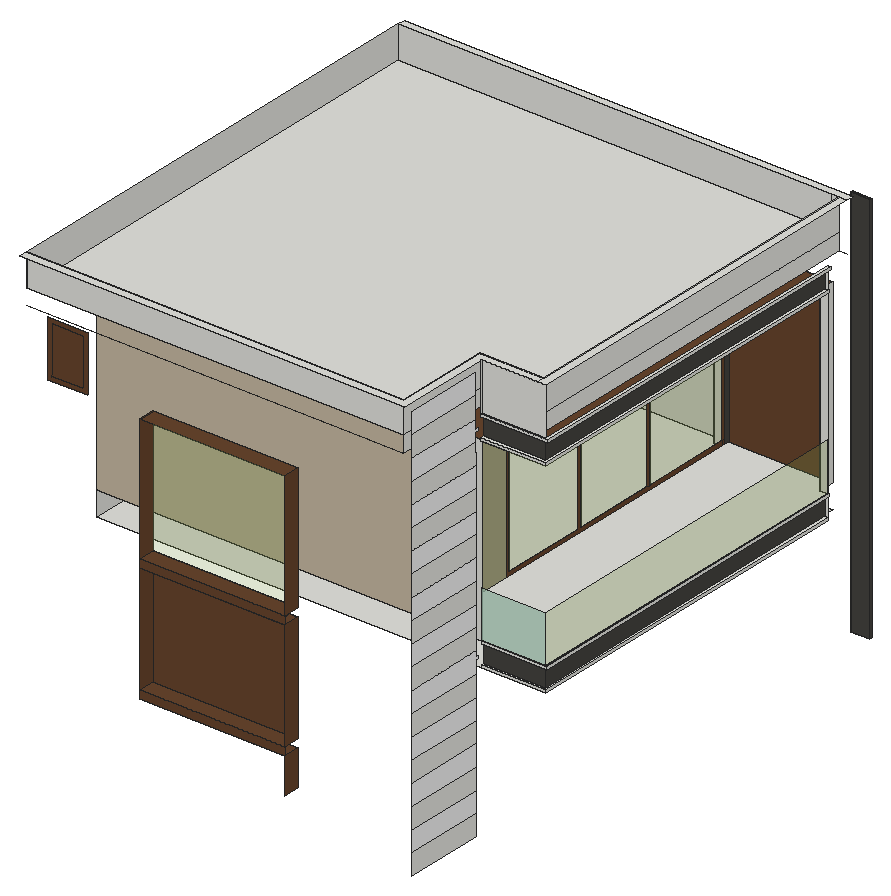
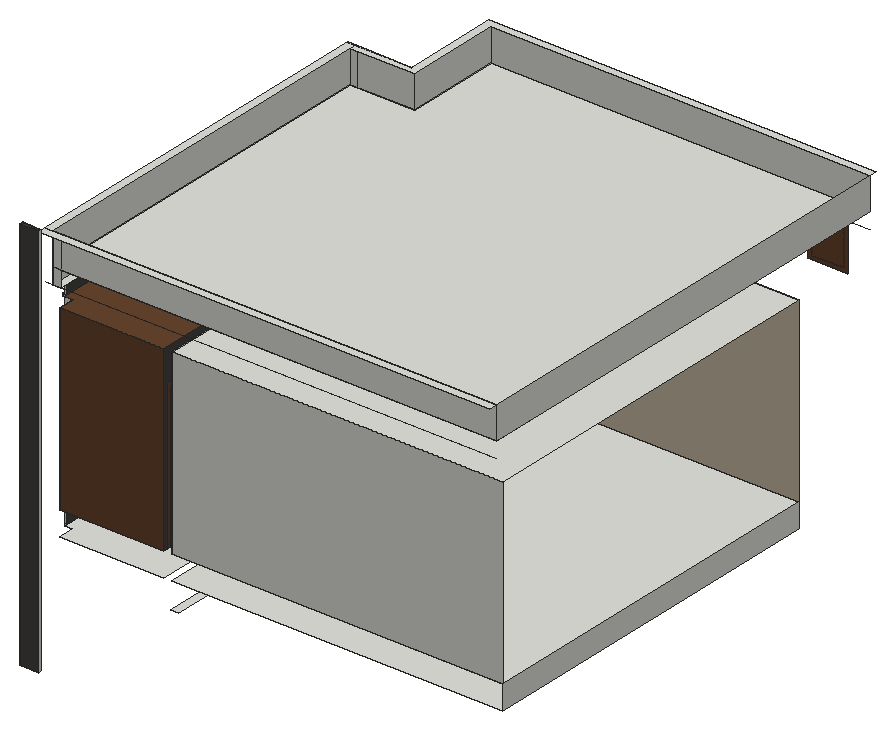
# SketchUp Ruby script. Lengths in inches.
U = 1.inch
M = Sketchup.active_model
def pt(a) = Geom::Point3d.new(a.map { |v| v * U })
def face(e, loops, mat)
  f = e.add_face(loops[0].map { |a| pt(a) })
  loops[1..].each { |l| e.add_face(l.map { |a| pt(a) }).erase! }
  f.material = f.back_material = mat if mat
  f
end
# faces: each face lists its corners as indices into pts; further lists are holes
def faces(e, pts, list, mat = nil) = list.each { |f| face(e, (f[0].is_a?(Array) ? f : [f]).map { |l| l.map { |i| pts[i] } }, mat) }
# xy, xz, yz: faces in a plane at the given z, y or x. An outline is a flat list of corners, or four numbers for a rectangle; further outlines are holes
def ring(l) = l.size == 4 ? [[l[0], l[1]], [l[2], l[1]], [l[2], l[3]], [l[0], l[3]]] : l.each_slice(2).to_a
def flat(e, list, mat, &to3) = list.each { |f| face(e, (f[0].is_a?(Array) ? f : [f]).map { |l| ring(l).map { |u, v| to3.(u, v) } }, mat) }
def xy(e, z, list, mat = nil) = flat(e, list, mat) { |x, y| [x, y, z] }
def xz(e, y, list, mat = nil) = flat(e, list, mat) { |x, z| [x, y, z] }
def yz(e, x, list, mat = nil) = flat(e, list, mat) { |y, z| [x, y, z] }
def lines(e, pts, list) = list.each { |a, b| e.add_line(pt(pts[a]), pt(pts[b])) }
# prism: a flat outline (further loops are holes) pulled along v
def prism(e, loops, v, mat = nil)
  f = face(e, loops, mat); d = Geom::Vector3d.new(v.map { |x| x * U })
  f.pushpull(f.normal.samedirection?(d) ? d.length : -d.length)
end
def box(e, o, s, mat = nil) = prism(e, [[o, [o[0] + s[0], o[1], o[2]], [o[0] + s[0], o[1] + s[1], o[2]], [o[0], o[1] + s[1], o[2]]]], [0, 0, s[2]], mat)
def at(x, y, z, deg = 0) = Geom::Transformation.translation(pt([x, y, z])) * Geom::Transformation.rotation(ORIGIN, Z_AXIS, deg.degrees)
def axes(o, x, y, z) = Geom::Transformation.new([*x, 0, *y, 0, *z, 0, *pt(o).to_a, 1])
def part(name) = M.definitions.add(name)
# library, detail: a bought-in or finely detailed component or shape, given as its bounding box
def library(name, o, s) = part(name).tap { |d| box(d.entities, o, s) }
def detail(e, o, s) = box(e.add_group.entities, o, s)
def put(e, d, t, mat = nil) = e.add_instance(d, t).tap { |i| i.material = mat if mat }
def group(e, t, mat = nil) = e.add_group.tap { |g| g.transformation = t; g.material = mat if mat }.entities
root = M.entities
M.materials.add("Carpet_2_1K").color = [170, 169, 131]
M.materials.add("Glass_Basic_1").color = [156, 186, 90]
M.materials["Glass_Basic_1"].alpha = 0.25
M.materials.add("LightPink_Translucent").color = [175, 214, 192]
M.materials["LightPink_Translucent"].alpha = 0.75
M.materials.add("ThomThom - Beard1").color = [198, 185, 162]
M.materials.add("Wood_Planks_01_1K").color = [69, 67, 63]
M.materials.add("Wood_Veneer_15_1K").color = [103, 69, 45]
M.materials.add("[0133_Gray]").color = [239, 239, 239]
xy(root,169.19,[[412,606,426,608]])
xy(root,196,[[167.51,246,276,258]],"Wood_Veneer_15_1K")
xy(root,202.12,[[167.51,246,276,258]],"Wood_Veneer_15_1K")
xy(root,231,[[324,318,330,588]])
xy(root,255,[[77.51,318,324,594],[330,318,330,594,408,594,408,582,414,582,414,318]])
xy(root,257,[[366,318,412,320],[412,318,414,582]])
xy(root,271,[[366,318,412,320],[412,318,414.78,582]])
xy(root,273,[[77.51,318,330,318,330,588,324,588,324,594,77.51,594],[330,318,414,318,414,582,408,582,408,594,330,594],[414,318,414.78,582]])
xy(root,284,[[167.51,246,173.51,258],[173.51,246,270,258],[270,246,276,258]],"Wood_Veneer_15_1K")
xy(root,290,[[167.51,246,276,258]],"Wood_Veneer_15_1K")
xy(root,384,[[324,318,330,588]])
xy(root,384,[[167.51,246,276,258]],"Wood_Veneer_15_1K")
xy(root,408,[[77.51,318,324,594]])
xy(root,408,[[366,317.22,366,318,330,318,330,594,408,594,408,582,414.78,582,414.78,317.22]],"Wood_Veneer_15_1K")
xy(root,410,[[366,317.22,412,320],[412,317.22,414.78,582]])
xy(root,424,[[366,317.22,412,320],[412,317.22,416,582]])
xy(root,426,[[366,317.22,408,318],[408,317.22,414,318],[414,317.22,416,582],[402,323.22,408,600]])
xy(root,438,[[77.51,252,360,252,360,323.22,408,323.22,408,600,77.51,600]])
xy(root,462,[[77.51,246,366,246,366,318,408,318,408,323.22,360,323.22,360,252,77.51,252],[408,318,414,600],[77.51,600,414,606]])
xy(root,464,[[412,606,426,608]],"Wood_Planks_01_1K")
xz(root,246,[[167.51,196,276,202.12],[167.51,284,276,290],[[98.48,386.35,128.48,428.35],[101.48,389.35,125.48,425.35]],[101.48,389.35,125.48,425.35]],"Wood_Veneer_15_1K")
xz(root,252,[[77.51,438,360,462]])
xz(root,258,[[167.51,290,276,384]],"Glass_Basic_1")
xz(root,258,[[167.51,202.12,276,284]],"Wood_Veneer_15_1K")
xz(root,317.22,[[366,408,414.78,410],[366,424,416,426]])
xz(root,318,[[324,144,330,231],[366,255,414,257],[366,271,414.78,273],[324,273,330,384],[330,273,366,408],
  [366,426,414,462]])
xz(root,318,[[366,273,414,309]],"LightPink_Translucent")
xz(root,318,[[77.51,273,324,408]],"ThomThom - Beard1")
xz(root,320,[[366,257,412,271],[366,410,412,424]],"Wood_Planks_01_1K")
xz(root,323.22,[[360,426,402,438],[402,426,408,438],[360,438,402,462],[402,438,408,462]])
xz(root,582,[[412,257,414,271],[414,271,414.78,273],[408,273,414,408],[414,408,414.78,410],[412,410,414,424],
  [414,424,416,426]])
xz(root,588,[[324,273,330,384]])
xz(root,594,[[77.51,273,324,408]])
xz(root,594,[[330,273,408,408]],"Wood_Veneer_15_1K")
xz(root,600,[[402,426,408,438],[77.51,438,402,462],[402,438,408,462]])
xz(root,606,[[412,169.19,426,464]],"Wood_Planks_01_1K")
xz(root,608,[[412,169.19,426,464]],"Wood_Planks_01_1K")
yz(root,77.51,[[318,255,594,273],[252,438,600,462]])
yz(root,167.51,[[246,202.12,258,284],[246,290,258,384]],"Wood_Veneer_15_1K")
yz(root,276,[[246,169.19,258,196],[246,202.12,258,284],[246,290,258,384]],"Wood_Veneer_15_1K")
yz(root,324,[[588,273,588,384,318,384,318,408,594,408,594,273]])
yz(root,330,[[318,273,385.5,384]],"Carpet_2_1K")
yz(root,330,[[388.5,276,453,381],[456,276,517.5,381],[520.5,276,588,381]],"Glass_Basic_1")
yz(root,330,[[591,273,594,273,594,408,318,408,318,384,591,384]],"Wood_Planks_01_1K")
yz(root,330,[[385.5,273,588,273,588,276,456,276,456,381,453,381,453,276,388.5,276,388.5,381,385.5,381],[588,273,591,276],[517.5,276,520.5,381],[588,276,591,384],[385.5,381,388.5,384],
  [388.5,381,453,384],[453,381,456,384],[456,381,517.5,384],[517.5,381,520.5,384],[520.5,381,588,384]],"Wood_Veneer_15_1K")
yz(root,360,[[252,426,323.22,438],[252,438,323.22,462]])
yz(root,366,[[252,144,312,159.6],[252,175.2,312,190.8],[252,206.4,312,222],[252,237.6,312,253.2],[252,268.8,312,284.4],
  [252,300,312,315.6],[252,331.2,312,346.8],[252,362.4,312,378],[252,393.6,312,393.6,312,402,311.22,402,311.22,409.2,252,409.2],[252,424.8,311.22,440.4],
  [317.22,426,318,462]])
yz(root,366,[[252,159.6,312,175.2],[252,190.8,312,206.4],[252,222,312,237.6],[252,253.2,312,253.2,312,263,314,263,314,265,312,265,312,268.8,252,268.8],[252,284.4,312,300],
  [252,315.6,312,331.2],[252,346.8,312,362.4],[252,378,312,393.6],[252,409.2,311.22,409.2,311.22,416,314,416,314,418,311.22,418,311.22,424.8,252,424.8],[252,440.4,311.22,456]],"[0133_Gray]")
yz(root,408,[[582,273,594,408],[323.22,426,600,438],[323.22,438,600,462]])
yz(root,412,[[606,169.19,608,464]])
yz(root,412,[[320,257,582,271],[320,410,582,424]],"Wood_Planks_01_1K")
yz(root,414,[[318,255,582,257]])
yz(root,414,[[318,273,582,309]],"Glass_Basic_1")
yz(root,414.78,[[318,271,582,273],[317.22,408,582,410]])
yz(root,416,[[317.22,424,582,426]])
yz(root,426,[[606,169.19,608,464]],"Wood_Planks_01_1K")
p = [[408,600,426],[414,600,426],[77.51,252,426],[360,252,426],[402,600,426],[77.51,600,426]]
lines(root,p,[[0,1],[2,3],[4,5]])
